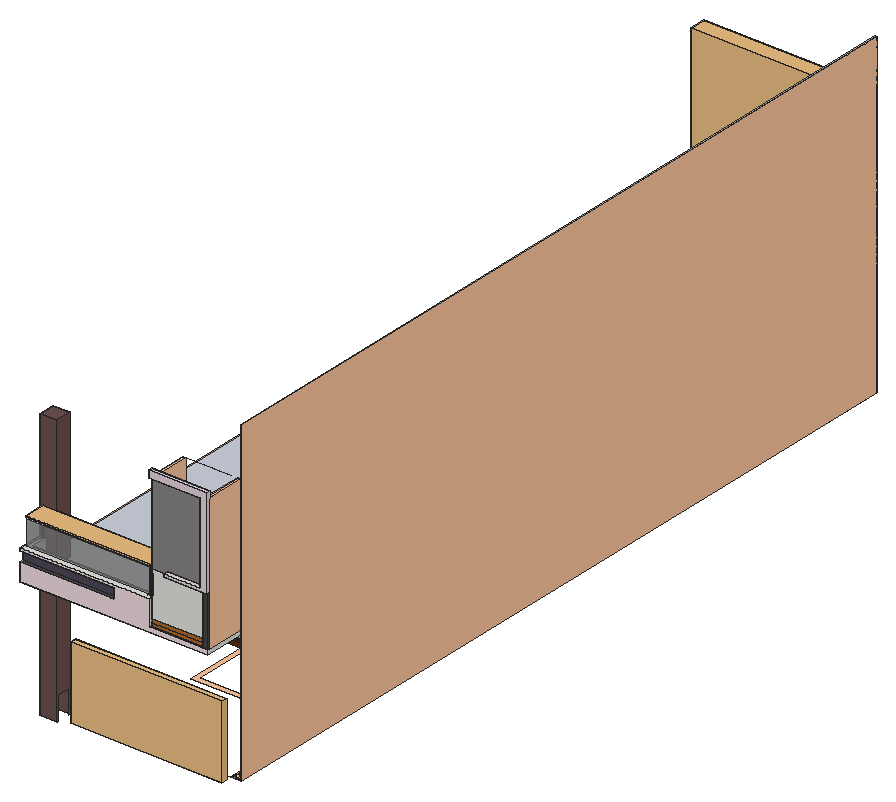
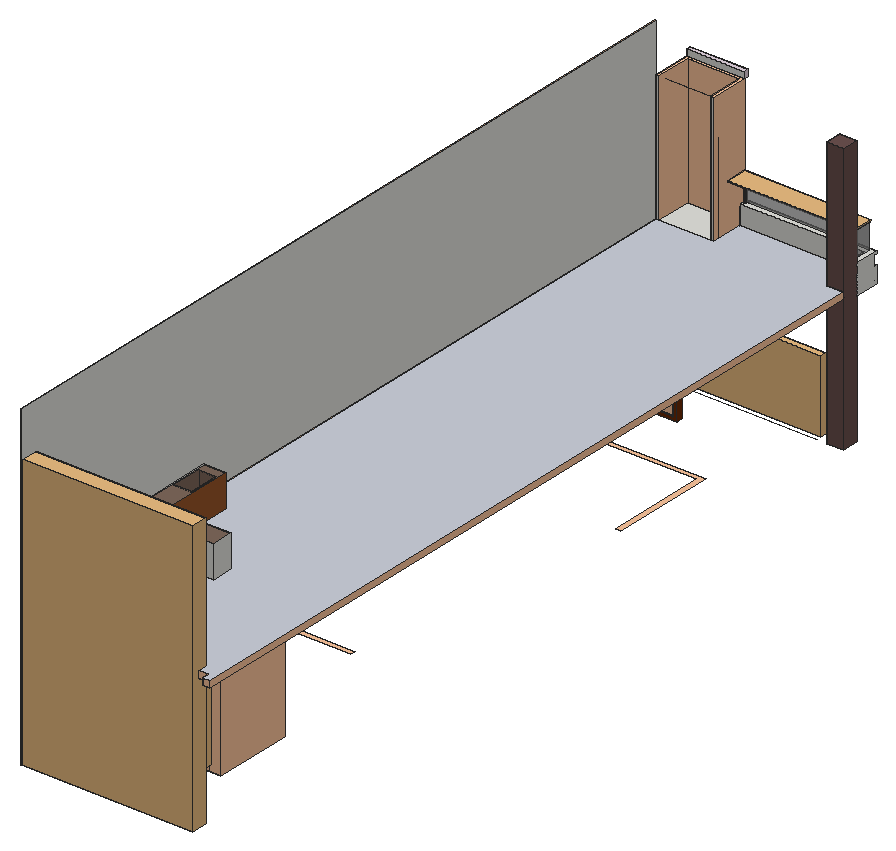
# SketchUp Ruby script. Lengths in inches.
U = 1.inch
M = Sketchup.active_model
def pt(a) = Geom::Point3d.new(a.map { |v| v * U })
def face(e, loops, mat)
  f = e.add_face(loops[0].map { |a| pt(a) })
  loops[1..].each { |l| e.add_face(l.map { |a| pt(a) }).erase! }
  f.material = f.back_material = mat if mat
  f
end
# faces: each face lists its corners as indices into pts; further lists are holes
def faces(e, pts, list, mat = nil) = list.each { |f| face(e, (f[0].is_a?(Array) ? f : [f]).map { |l| l.map { |i| pts[i] } }, mat) }
# xy, xz, yz: faces in a plane at the given z, y or x. An outline is a flat list of corners, or four numbers for a rectangle; further outlines are holes
def ring(l) = l.size == 4 ? [[l[0], l[1]], [l[2], l[1]], [l[2], l[3]], [l[0], l[3]]] : l.each_slice(2).to_a
def flat(e, list, mat, &to3) = list.each { |f| face(e, (f[0].is_a?(Array) ? f : [f]).map { |l| ring(l).map { |u, v| to3.(u, v) } }, mat) }
def xy(e, z, list, mat = nil) = flat(e, list, mat) { |x, y| [x, y, z] }
def xz(e, y, list, mat = nil) = flat(e, list, mat) { |x, z| [x, y, z] }
def yz(e, x, list, mat = nil) = flat(e, list, mat) { |y, z| [x, y, z] }
def lines(e, pts, list) = list.each { |a, b| e.add_line(pt(pts[a]), pt(pts[b])) }
# prism: a flat outline (further loops are holes) pulled along v
def prism(e, loops, v, mat = nil)
  f = face(e, loops, mat); d = Geom::Vector3d.new(v.map { |x| x * U })
  f.pushpull(f.normal.samedirection?(d) ? d.length : -d.length)
end
def box(e, o, s, mat = nil) = prism(e, [[o, [o[0] + s[0], o[1], o[2]], [o[0] + s[0], o[1] + s[1], o[2]], [o[0], o[1] + s[1], o[2]]]], [0, 0, s[2]], mat)
def at(x, y, z, deg = 0) = Geom::Transformation.translation(pt([x, y, z])) * Geom::Transformation.rotation(ORIGIN, Z_AXIS, deg.degrees)
def axes(o, x, y, z) = Geom::Transformation.new([*x, 0, *y, 0, *z, 0, *pt(o).to_a, 1])
def part(name) = M.definitions.add(name)
# library, detail: a bought-in or finely detailed component or shape, given as its bounding box
def library(name, o, s) = part(name).tap { |d| box(d.entities, o, s) }
def detail(e, o, s) = box(e.add_group.entities, o, s)
def put(e, d, t, mat = nil) = e.add_instance(d, t).tap { |i| i.material = mat if mat }
def group(e, t, mat = nil) = e.add_group.tap { |g| g.transformation = t; g.material = mat if mat }.entities
root = M.entities
M.materials.add("[Brick Tumbled]").color = [135, 132, 132]
M.materials.add("[Color A01]").color = [243, 201, 104]
M.materials.add("[Color A02]1").color = [252, 197, 157]
M.materials.add("[Color A02]3").color = [226, 211, 222]
M.materials.add("[Color B01]").color = [107, 81, 79]
M.materials.add("[Color B06]").color = [239, 219, 223]
M.materials.add("[Color M06]").color = [77, 72, 86]
M.materials.add("[Granite Brown]").color = [126, 104, 91]
M.materials.add("[Granite Dark Gray]").color = [69, 68, 68]
M.materials.add("[Marble Carrara Floor Tile]").color = [204, 208, 219]
M.materials.add("[Metal Aluminum Anodized]").color = [202, 209, 219]
M.materials.add("[Tile Veriegated Stone]").color = [171, 137, 112]
M.materials.add("[Translucent Glass Gray]1").color = [132, 132, 132]
M.materials["[Translucent Glass Gray]1"].alpha = 0.5
M.materials.add("[Wood Bamboo]").color = [177, 105, 43]
M.materials.add("[Wood Cherry Original]").color = [152, 86, 42]
M.materials.add("[Wood Fence]").color = [130, 51, 1]
M.materials.add("[Wood Veneer 02]").color = [107, 42, 7]
c1 = library("Group\#155",[-46.99,0,0],[159.06,15.07,255.07])
c2 = library("Slatted double gate",[-0.09,68.76,-0.1],[107.6,5.32,60.06])
c3 = library("Group\#179",[-0.01,-1.53,0.79],[112.05,69.48,120])
c4 = part("Group222\#1")
xy(c4.entities,0,[[[-24,-24,24,24],[-20.4375,-20.4375,-7.1,20.4375],[-6.67,-20.4375,6.67,20.4375],[7.1,-20.4375,20.4375,20.4375]]],"[Wood Veneer 02]")
xy(c4.entities,0.375,[[-20.4375,-20.4375,-20.0625,-20.0625,-7.48,-20.0625,-7.1,-20.4375],[-20.4375,-20.4375,-20.4375,20.4375,-20.0625,20.0625,-20.0625,-20.0625],[-7.1,-20.4375,-7.48,-20.0625,-7.48,20.0625,-7.1,20.4375],[-6.67,-20.4375,-6.29,-20.0625,6.29,-20.0625,6.67,-20.4375],[-6.67,-20.4375,-6.67,20.4375,-6.29,20.0625,-6.29,-20.0625],
  [6.67,-20.4375,6.29,-20.0625,6.29,20.0625,6.67,20.4375],[7.1,-20.4375,7.1,20.4375,7.48,20.0625,7.48,-20.0625],[7.1,-20.4375,7.48,-20.0625,20.0625,-20.0625,20.4375,-20.4375],[20.4375,-20.4375,20.0625,-20.0625,20.0625,20.0625,20.4375,20.4375],[-20.0625,20.0625,-20.4375,20.4375,-7.1,20.4375,-7.48,20.0625],
  [-6.29,20.0625,-6.67,20.4375,6.67,20.4375,6.29,20.0625],[7.48,20.0625,7.1,20.4375,20.4375,20.4375,20.0625,20.0625]],"[Wood Veneer 02]")
xy(c4.entities,5.5,[[-20.4375,-20.4375,-20.0625,-20.0625,-20.0625,20.0625,-20.4375,20.4375],[-20.4375,-20.4375,-7.1,-20.4375,-7.48,-20.0625,-20.0625,-20.0625],[-7.1,-20.4375,-7.1,20.4375,-7.48,20.0625,-7.48,-20.0625],[-6.67,-20.4375,-6.29,-20.0625,-6.29,20.0625,-6.67,20.4375],[-6.67,-20.4375,6.67,-20.4375,6.29,-20.0625,-6.29,-20.0625],
  [6.67,-20.4375,6.67,20.4375,6.29,20.0625,6.29,-20.0625],[7.1,-20.4375,20.4375,-20.4375,20.0625,-20.0625,7.48,-20.0625],[7.1,-20.4375,7.48,-20.0625,7.48,20.0625,7.1,20.4375],[20.4375,-20.4375,20.4375,20.4375,20.0625,20.0625,20.0625,-20.0625],[-20.0625,20.0625,-7.48,20.0625,-7.1,20.4375,-20.4375,20.4375],
  [-6.29,20.0625,6.29,20.0625,6.67,20.4375,-6.67,20.4375],[7.48,20.0625,20.0625,20.0625,20.4375,20.4375,7.1,20.4375]],"[Wood Veneer 02]")
xy(c4.entities,5.875,[[[-24,-24,24,24],[-20.4375,-20.4375,-7.1,20.4375],[-6.67,-20.4375,6.67,20.4375],[7.1,-20.4375,20.4375,20.4375]]],"[Wood Veneer 02]")
xz(c4.entities,-24,[[-24,0,24,5.875]],"[Wood Veneer 02]")
xz(c4.entities,-20.4375,[[-20.4375,0,-7.1,0.375],[-6.67,0,6.67,0.375],[7.1,0,20.4375,0.375],[-20.4375,5.5,-7.1,5.875],[-6.67,5.5,6.67,5.875],
  [7.1,5.5,20.4375,5.875]],"[Wood Veneer 02]")
xz(c4.entities,-20.0625,[[-20.0625,0.375,-7.48,5.5],[-6.29,0.375,6.29,5.5],[7.48,0.375,20.0625,5.5]],"[Wood Veneer 02]")
xz(c4.entities,20.0625,[[-20.0625,0.375,-7.48,5.5],[-6.29,0.375,6.29,5.5],[7.48,0.375,20.0625,5.5]],"[Wood Veneer 02]")
xz(c4.entities,20.4375,[[-20.4375,0,-7.1,0.375],[-6.67,0,6.67,0.375],[7.1,0,20.4375,0.375],[-20.4375,5.5,-7.1,5.875],[-6.67,5.5,6.67,5.875],
  [7.1,5.5,20.4375,5.875]],"[Wood Veneer 02]")
xz(c4.entities,24,[[-24,0,24,5.875]],"[Wood Veneer 02]")
yz(c4.entities,-24,[[-24,0,24,5.875]],"[Wood Veneer 02]")
yz(c4.entities,-20.4375,[[-20.4375,0,20.4375,0.375],[-20.4375,5.5,20.4375,5.875]],"[Wood Veneer 02]")
yz(c4.entities,-20.0625,[[-20.0625,0.375,20.0625,5.5]],"[Wood Veneer 02]")
yz(c4.entities,-7.48,[[-20.0625,0.375,20.0625,5.5]],"[Wood Veneer 02]")
yz(c4.entities,-7.1,[[-20.4375,0,20.4375,0.375],[-20.4375,5.5,20.4375,5.875]],"[Wood Veneer 02]")
yz(c4.entities,-6.67,[[-20.4375,0,20.4375,0.375],[-20.4375,5.5,20.4375,5.875]],"[Wood Veneer 02]")
yz(c4.entities,-6.29,[[-20.0625,0.375,20.0625,5.5]],"[Wood Veneer 02]")
yz(c4.entities,6.29,[[-20.0625,0.375,20.0625,5.5]],"[Wood Veneer 02]")
yz(c4.entities,6.67,[[-20.4375,0,20.4375,0.375],[-20.4375,5.5,20.4375,5.875]],"[Wood Veneer 02]")
yz(c4.entities,7.1,[[-20.4375,0,20.4375,0.375],[-20.4375,5.5,20.4375,5.875]],"[Wood Veneer 02]")
yz(c4.entities,7.48,[[-20.0625,0.375,20.0625,5.5]],"[Wood Veneer 02]")
yz(c4.entities,20.0625,[[-20.0625,0.375,20.0625,5.5]],"[Wood Veneer 02]")
yz(c4.entities,20.4375,[[-20.4375,0,20.4375,0.375],[-20.4375,5.5,20.4375,5.875]],"[Wood Veneer 02]")
yz(c4.entities,24,[[-24,0,24,5.875]],"[Wood Veneer 02]")
c5 = part("Round rod")
prism(c5.entities,[[[1.59,1.03,0],[1.625,0.82,0],[1.6,0.61,0],[1.52,0.42,0],[1.4,0.25,0],[1.23,0.11,0],[1.03,0.03,0],[0.82,0,0],[0.61,0.02,0],[0.42,0.1,0],[0.25,0.23,0],[0.11,0.4,0],[0.03,0.59,0],[0,0.8,0],[0.02,1.01,0],[0.1,1.21,0],[0.23,1.38,0],[0.4,1.51,0],[0.59,1.59,0],[0.8,1.625,0],[1.01,1.6,0],[1.21,1.52,0],[1.38,1.4,0],[1.51,1.23,0]]],[0,0,25.375])
c6 = part("Component\#5")
box(c6.entities,[0,-0.625,0],[48.6875,0.625,3.09])
xy(root,-0.11,[[[166.9,46.0625,175.89,46.0625,175.89,61,171.33,61,171.33,61.13,166.9,61.13],[167.91,47.08,167.91,49.86,168.54,49.23,167.91,48.6,167.91,48.09,168.54,47.46,168.17,47.08,168.93,47.08,168.54,47.46,169.42,48.35,170.32,47.46,169.94,47.08,170.7,47.08,170.32,47.46,171.19,48.36,172.09,47.46,171.71,47.08,172.47,47.08,172.09,47.46,172.95,48.37,172.07,49.26,172.94,50.15,172.06,51.04,171.18,50.14,170.3,51.02,169.42,50.13,170.3,49.25,169.42,48.35,168.54,49.23,169.42,50.13,168.54,51.01,169.42,51.9,168.54,52.78,169.42,53.67,168.54,54.55,167.91,53.91,167.91,53.41,168.54,52.78,167.91,52.14,167.91,58.73,168.55,58.09,169.43,58.98,168.29,60.12,172.35,60.12,170.32,58.09,169.43,58.98,168.55,58.09,169.43,57.21,168.55,56.32,170.3,54.57,171.18,55.46,172.06,56.36,172.93,55.48,173.8125,56.37,172.93,57.25,173.8125,58.15,174.69,59.04,173.8,59.93,173.99,60.12,174.88,60.12,174.88,59.23,174.69,59.04,173.8125,58.15,174.69,57.27,173.8125,56.37,174.69,55.49,174.88,55.31,174.88,53.91,174.69,53.72,173.8125,52.83,172.93,51.93,173.82,51.05,174.69,50.17,172.95,48.37,173.85,47.47,173.49,47.08],[174.88,57.08,174.69,57.27,174.88,57.46],[174.88,48.22,174.7,48.4,174.88,48.6]],[167.91,47.08,168.17,47.08,168.54,47.46,167.91,48.09],[168.93,47.08,169.94,47.08,170.32,47.46,169.42,48.35,168.54,47.46],[170.7,47.08,171.71,47.08,172.09,47.46,171.19,48.36,170.32,47.46],[172.47,47.08,173.49,47.08,173.85,47.47,172.95,48.37,172.09,47.46],
  [174.25,47.08,174.88,47.08,174.88,48.22,174.7,48.4,173.85,47.47],[174.88,48.22,174.88,48.6,174.7,48.4],[167.91,48.6,168.54,49.23,167.91,49.86],[174.88,49.99,174.88,50.37,174.69,50.17],[167.91,50.37,168.54,51.01,167.91,51.63],
  [174.88,51.76,174.88,52.14,174.69,51.95],[171.18,51.92,172.06,52.8125,172.93,53.71,170.3,56.34,169.42,55.45,168.55,56.32,167.91,55.6875,167.91,55.18,169.42,53.67,170.3,52.8],[167.91,52.14,168.54,52.78,167.91,53.41],[174.69,53.72,174.88,53.91,174.88,55.31,174.69,55.49,173.8125,54.6],[167.91,53.91,168.54,54.55,167.91,55.18],
  [167.91,55.6875,168.55,56.32,167.91,56.95],[168.55,56.32,167.91,56.95,167.91,57.46,168.55,58.09,170.3,56.34,171.17,57.24,170.32,58.09,169.43,57.21],[174.88,57.08,174.88,57.46,174.69,57.27],[167.91,57.46,168.55,58.09,167.91,58.73],[174.69,59.04,174.88,59.23,174.88,60.12,173.99,60.12,173.8,59.93],
  [168.55,59.86,168.8,60.12,168.29,60.12],[170.32,59.86,170.57,60.12,170.07,60.12],[172.09,59.86,172.35,60.12,171.84,60.12],[171.33,61,175.89,61.13],[171.33,61.13,171.33,142.17,142.65,142.17,141.07,143.82,140.6875,143.4375,142.01,142.17,52.81,142.17,52.81,241.2,57.37,241.2,57.37,146.61,171.33,146.61,171.33,212.2,175.89,212.2,175.89,61.13],
  [142.01,142.17,140.6875,143.4375,141.07,143.82,142.65,142.17],[166.9,212.2,171.33,212.2,171.33,213.21,167.91,213.21,167.91,226.13,171.33,226.13,171.33,227.14,166.9,227.14],[171.33,212.2,175.89,212.2,175.89,227.14,171.33,227.14,171.33,226.13,174.88,226.13,174.88,213.21,171.33,213.21],[167.91,213.21,168.17,213.21,168.55,213.59,167.91,214.22],[168.17,213.21,168.93,213.21,168.55,213.59],
  [168.93,213.21,169.94,213.21,170.32,213.59,169.43,214.48,168.55,213.59],[169.94,213.21,170.7,213.21,170.32,213.59],[170.7,213.21,171.33,213.21,171.33,214.35,171.21,214.48,170.32,213.59],[171.33,213.21,171.71,213.21,172.09,213.59,171.33,214.35],[172.47,213.21,173.49,213.21,173.87,213.59,172.98,214.48,172.09,213.59],
  [170.32,213.59,171.21,214.48,170.32,215.36,169.43,214.48],[174.88,214.22,174.88,214.6,174.69,214.42],[174.69,214.42,174.88,214.6,174.88,216,174.69,216.1875,173.8125,215.3125],[171.33,214.6,172.09,215.36,171.33,216.125],[171.33,216.125,171.33,216.38,171.21,216.25],
  [171.33,216.38,172.06,217.1,171.33,217.83],[172.06,217.1,172.93,217.98,172.06,218.87,171.33,218.15,171.33,217.83],[171.33,217.83,171.33,218.15,171.18,217.99],[169.43,218.02,170.3,218.89,169.42,219.78,168.55,218.91],[171.33,218.15,172.06,218.87,171.33,219.61],
  [172.06,218.87,172.92,219.73,172.03,220.62,171.33,219.92,171.33,219.61],[170.3,218.89,171.18,219.77,170.3,220.66,169.42,219.78],[171.33,219.61,171.33,219.92,171.18,219.77],[169.42,219.78,170.3,220.66,169.42,221.56,168.54,220.68],[172.03,220.62,172.92,221.51,172.03,222.39,171.33,221.7,171.33,221.32],
  [173.8,220.62,174.6875,221.51,173.8,222.39,172.92,221.51],[170.3,220.66,171.14,221.51,170.26,222.39,169.42,221.56],[171.33,221.32,171.33,221.7,171.14,221.51],[171.14,221.51,171.33,221.7,171.33,223.09,171.14,223.28,170.26,222.39],[172.92,221.51,173.8,222.39,172.92,223.28,172.03,222.39],
  [172.03,222.39,172.92,223.28,172.03,224.16,171.33,223.47,171.33,223.09],[173.8,222.39,174.6875,223.28,173.8,224.16,172.92,223.28],[171.33,223.09,171.33,223.47,171.14,223.28],[169.39,223.26,170.29,224.13,169.41,225.02,168.5,224.15],[172.92,223.28,173.8,224.16,172.92,225.05,172.03,224.16],
  [167.91,223.6,168.5,224.15,167.91,224.73],[170.29,224.13,171.19,225,170.3125,225.88,169.41,225.02],[168.5,224.15,169.41,225.02,168.53,225.89,167.91,225.37,167.91,224.73],[173.8,224.16,174.6875,225.05,173.8,225.9375,172.92,225.05],[168.17,372.26,168.93,372.26,168.55,372.64],
  [171.33,372.26,171.71,372.26,172.09,372.64,171.33,373.4],[171.71,372.26,172.47,372.26,172.09,372.64],[169.43,373.52,170.32,374.41,169.43,375.3,168.55,374.41],[170.32,374.41,171.21,375.3,170.32,376.18,169.43,375.3],[169.43,375.3,170.32,376.18,169.43,377.07,168.55,376.18],
  [171.21,375.3,171.33,375.42,171.33,376.88,171.18,377.04,170.32,376.18],[170.32,376.18,171.18,377.04,170.3,377.93,169.43,377.07],[174.88,376.82,174.88,377.19,174.69,377.01],[174.69,377.01,174.88,377.19,174.88,378.59,174.69,378.78,173.8125,377.9],[169.43,377.07,170.3,377.93,169.42,378.83,168.55,377.95],
  [170.3,377.93,171.18,378.8125,170.3,379.71,169.42,378.83],[174.69,378.78,174.88,378.97,174.88,380.36,174.69,380.55,173.8125,379.67],[169.42,378.83,170.3,379.71,169.4,380.62,168.53,379.73],[170.3,379.71,171.18,380.58,170.27,381.5,169.4,380.62],[174.69,380.55,174.88,380.74,174.88,382.13,174.69,382.33,173.82,381.45],
  [169.4,380.62,170.27,381.5,169.42,382.37,168.54,381.49],[170.27,381.5,171.15,382.39,170.3,383.25,169.42,382.37],[172.94,382.35,173.82,383.23,172.9,384.1875,172.02,383.29],[169.42,382.37,170.3,383.25,169.42,384.15,168.54,383.27],[173.82,383.23,174.7,384.11,173.8,385.1,172.9,384.1875],
  [170.3,383.25,171.19,384.14,170.32,385.04,169.42,384.15],[173.8,385.1,173.99,385.3,173.61,385.3],[171.33,386.1875,171.33,501.8,92.32,501.8,92.32,506.23,171.33,506.23,171.33,563.34,175.89,563.34,175.89,386.1875],[166.9,563.34,175.89,563.34,175.89,578.28,171.33,578.28,171.33,577.27,174.88,577.27,174.88,564.35,167.91,564.35,167.91,577.27,171.33,577.27,171.33,578.28,166.9,578.28],[167.91,564.35,168.17,564.35,168.55,564.73,167.91,565.36],
  [168.17,564.35,168.93,564.35,168.55,564.73,169.43,565.62,168.55,566.5,167.91,565.87,167.91,565.36,168.55,564.73],[169.94,564.35,170.7,564.35,170.32,564.73],[171.71,564.35,172.47,564.35,172.09,564.73],[172.47,564.35,173.49,564.35,173.87,564.73,172.98,565.62,172.09,564.73],[173.49,564.35,174.25,564.35,173.87,564.73],
  [174.25,564.35,174.88,564.35,174.88,565.36,174.69,565.56,173.87,564.73],[168.55,564.73,169.43,565.62,168.55,566.5,167.91,565.87,167.91,565.36],[172.09,564.73,172.98,565.62,172.09,566.5,171.21,565.62],[171.21,565.62,172.09,566.5,171.21,567.39,170.32,566.5],[167.91,565.87,168.55,566.5,167.91,567.14],
  [168.55,566.5,169.43,567.39,168.55,568.28,167.91,567.64,167.91,567.14],[172.09,566.5,172.93,567.34,172.06,568.24,171.21,567.39],[167.91,567.64,168.55,568.28,167.91,568.91],[168.55,568.28,169.43,569.16,168.55,570.05,167.91,569.42,167.91,568.91],[174.88,568.91,174.88,569.29,174.6875,569.1],
  [171.33,568.97,171.33,569.29,171.18,569.13],[174.6875,569.1,174.88,569.29,174.88,570.68,174.6875,570.87,173.8,569.99],[173.8,571.76,174.6875,572.65,173.8,573.53,172.92,572.65],[172.92,572.65,173.8,573.53,172.92,574.42,172.03,573.53],[172.03,573.53,172.92,574.42,172.03,575.3,171.33,574.61,171.33,574.23],
  [173.8,573.53,174.6875,574.42,173.8,575.3,172.92,574.42],[171.33,574.23,171.33,574.61,171.14,574.42],[174.88,574.23,174.88,574.61,174.6875,574.42],[172.92,574.42,173.8,575.3,172.92,576.19,172.03,575.3],[172.03,575.3,172.92,576.19,172.09,577.02,171.33,576.28,171.33,576],
  [173.8,575.3,174.6875,576.19,173.8,577.08,172.92,576.19],[172.92,576.19,173.8,577.08,173.61,577.27,172.35,577.27,172.09,577.02],[174.6875,576.19,174.88,576.38,174.88,577.27,173.99,577.27,173.8,577.08],[171.33,576.28,172.09,577.02,171.84,577.27,171.33,577.27],[172.09,577.02,172.35,577.27,171.84,577.27],
  [173.8,577.08,173.99,577.27,173.61,577.27],[171.33,578.28,175.89,578.28,175.89,706.3,52.81,706.3,52.81,632.35,57.37,632.35,57.37,637.29,69.4,637.29,69.4,641.85,57.37,641.85,57.37,701.87,171.33,701.87],[89.4,637.29,171.33,641.85]],"[Color A02]1")
xy(root,0,[[175.91,46.0625,175.89,785.32,176.89,785.32,176.91,46.0625]])
xy(root,113.57,[[153.02,587.14,169.46,615.87]],"[Granite Brown]")
xy(root,125.89,[[0.89,46.0625,7.86,784.43],[171.33,61,175.89,61,175.89,212.2,171.33,212.2,171.33,146.61,57.37,146.61,57.37,241.2,52.81,241.2,52.81,142.17,142.01,142.17,140.6875,143.4375,141.07,143.82,142.65,142.17,171.33,142.17],[142.01,142.17,142.26,142.17,140.6875,143.4375],[142.26,142.17,142.65,142.17,141.07,143.82,140.6875,143.4375],[171.33,227.14,175.89,227.14,175.89,371.24,171.33,371.24,171.33,318.69,126.89,318.69,126.89,341.23,122.33,341.23,122.33,318.69,57.37,318.69,57.37,371.24,126.89,371.24,126.89,375.68,57.37,375.68,57.37,501.8,63.32,501.8,63.32,506.23,57.37,506.23,57.37,585.88,52.81,585.88,52.81,283.24,57.37,283.24,57.37,314.26,171.33,314.26],
  [171.33,386.1875,175.89,386.1875,175.89,563.34,171.33,563.34,171.33,506.23,92.32,506.23,92.32,501.8,171.33,501.8],[171.33,578.28,175.89,578.28,175.89,706.3,52.81,706.3,52.81,632.35,57.37,632.35,57.37,637.29,69.4,637.29,69.4,641.85,57.37,641.85,57.37,701.87,171.33,701.87]],"[Color A02]1")
xy(root,131.89,[[151.27,578.28,151.27,646.1,92.44,646.1,92.44,665.91,171.33,665.91,171.33,578.28]])
xy(root,161.89,[[[151.27,578.28,171.33,578.28,171.33,665.91,92.44,665.91,92.44,646.1,151.27,646.1],[153.02,587.14,169.46,615.87]]],"[Granite Brown]")
xy(root,297.2,[[175.91,46.0625,176.91,46.0625,176.89,785.32,175.89,785.32]])
xz(root,46.0625,[[175.91,0,176.91,297.2]])
xz(root,61,[[171.33,-0.11,175.89,125.89]],"[Color A02]1")
xz(root,146.61,[[75.18,41.89,123.18,89.89]],"[Color A02]1")
xz(root,212.2,[[166.89,125.89,175.89,125.9]],"[Color A02]1")
xz(root,227.14,[[166.89,125.89,175.89,125.9]],"[Color A02]1")
xz(root,371.25,[[166.89,125.89,175.89,125.9]],"[Color A02]1")
xz(root,386.1875,[[166.89,125.89,175.89,125.9]],"[Color A02]1")
xz(root,563.34,[[173.33,125.89,175.89,125.9]],"[Color A02]1")
xz(root,578.28,[[151.27,131.89,171.33,161.89]])
xz(root,578.28,[[171.33,-0.11,175.89,125.89],[166.7,125.89,166.9,125.9],[173.33,125.89,175.89,125.9]],"[Color A02]1")
xz(root,587.14,[[153.02,113.57,169.46,161.89]],"[Granite Brown]")
xz(root,615.87,[[153.02,113.57,169.46,161.89]],"[Granite Brown]")
xz(root,632.35,[[52.81,-0.11,57.37,125.89]],"[Color A02]1")
xz(root,637.29,[[57.37,-0.11,69.4,125.89]],"[Color A02]1")
xz(root,641.85,[[57.37,-0.11,69.4,125.89]],"[Color A02]1")
xz(root,646.1,[[92.44,131.89,151.27,161.89]],"[Wood Cherry Original]")
xz(root,665.91,[[92.44,131.89,171.33,161.89]])
xz(root,701.87,[[57.37,-0.11,171.33,0],[57.37,0,171.33,125.89],[171.33,0,171.91,125.89]],"[Color A02]1")
xz(root,706.3,[[52.81,-0.11,63.83,125.89],[63.83,-0.11,73.83,125.89],[73.83,-0.11,83.83,125.89],[83.83,-0.11,93.84,125.89],[93.84,-0.11,103.84,125.89],
  [103.84,-0.11,113.84,125.89],[113.84,-0.11,123.85,125.89],[123.85,-0.11,133.85,125.89],[133.85,-0.11,175.89,125.89]],"[Color A02]1")
xz(root,785.32,[[175.89,0,176.89,257.89],[175.89,257.89,176.89,297.2]])
yz(root,52.81,[[632.35,-0.11,706.3,125.89]],"[Color A02]1")
yz(root,57.37,[[632.35,-0.11,637.29,125.89],[641.85,-0.11,677.81,125.89],[677.81,-0.11,701.87,125.89]],"[Color A02]1")
yz(root,69.4,[[637.29,-0.11,641.85,125.89]],"[Color A02]1")
yz(root,92.44,[[646.1,131.89,665.91,161.89]])
yz(root,151.27,[[578.28,131.89,646.1,161.89]],"[Wood Cherry Original]")
yz(root,153.02,[[587.14,113.57,615.87,161.89]],"[Granite Brown]")
yz(root,166.89,[[212.2,125.89,227.14,125.9],[371.25,125.89,386.1875,125.9]],"[Color A02]1")
yz(root,169.46,[[587.14,113.57,615.87,161.89]],"[Granite Brown]")
yz(root,171.33,[[578.28,131.89,665.91,161.89]])
yz(root,171.33,[[61,-0.11,142.17,125.89],[578.28,-0.11,677.81,125.89],[677.81,-0.11,701.87,125.89]],"[Color A02]1")
yz(root,175.89,[[578.28,-0.11,706.3,125.89],[227.14,125.89,371.25,125.9],[386.1875,125.89,563.34,125.9]],"[Color A02]1")
p = [[175.89,785.32,257.89],[175.89,785.32,0],[175.91,46.0625,0],[175.91,46.0625,297.2],[175.89,785.32,297.2],[176.89,785.32,0],
  [176.89,785.32,257.89],[176.89,785.32,297.2],[176.91,46.0625,297.2],[176.91,46.0625,0],[25.85,46.0625,0],[166.9,46.0625,0],
  [166.9,61,121.89],[166.9,58.0625,121.89],[166.91,769.5,60],[166.91,769.76,60],[0.89,10.0625,125.89],[0.89,10.0625,125.9],
  [0.89,784.43,125.89],[0.89,784.43,125.9],[175.89,784.43,125.89],[175.89,784.43,125.9],[175.89,10.0625,125.89],[175.89,10.0625,125.9],
  [175.89,61,125.89],[175.89,46.0625,125.89],[92.89,146.61,45.82],[92.89,146.61,85.95],[79.12,146.61,85.95],[91.7,146.61,85.95],
  [79.12,146.61,45.82],[105.48,146.61,45.82],[91.7,146.61,45.82],[105.48,146.61,85.95],[106.66,146.61,45.82],[106.66,146.61,85.95],
  [119.25,146.61,45.82],[119.25,146.61,85.95],[91.7,145.11,45.82],[79.12,145.11,45.82],[79.12,145.11,85.95],[91.7,145.11,85.95],
  [105.48,145.11,45.82],[92.89,145.11,45.82],[92.89,145.11,85.95],[105.48,145.11,85.95],[119.25,145.11,45.82],[106.66,145.11,45.82],
  [106.66,145.11,85.95],[119.25,145.11,85.95]]
faces(root,p,[[0,1,2,3,4]])
faces(root,p,[[5,6,7,8,9]],"[Color A02]1")
lines(root,p,[[10,11],[12,13],[14,15],[16,17],[18,19],[20,21],[22,23],[24,25],[26,27],[28,29],[30,28],[31,26],
  [32,30],[27,33],[29,32],[33,31],[34,35],[36,34],[37,36],[35,37],[38,39],[39,40],[40,41],[41,38],
  [42,43],[43,44],[44,45],[45,42],[46,47],[47,48],[48,49],[49,46]])
put(root,c1,at(63.84,769.36,0))
g1 = group(root,at(0.89,30.95,0))
xy(g1,251.89,[[0,0,15.96,15.11]],"[Color B01]")
xz(g1,0,[[0,0,15.96,251.89]],"[Color B01]")
xz(g1,15.11,[[0,0,15.96,251.89]],"[Color B01]")
yz(g1,0,[[0,0,15.11,251.89]],"[Color B01]")
yz(g1,15.96,[[0,0,0.84,0,0.84,21.875,13.375,21.875,13.375,0,15.11,0,15.11,251.89,0,251.89]],"[Color B01]")
put(root,c2,axes([25.96,-33.09,0.11],[1.31104,0,0],[0,1,0],[0,0,1.1312]))
put(root,c3,at(62.29,707.83,5.1))
put(root,c4,axes([99.18,148.05,65.89],[1,0,0],[0,0,1],[0,-1,0]),"[Color A02]1")
g2 = group(root,at(0.89,46.0625,125.89))
xy(g2,-1.5625,[[26.98,-0.11,153.05,81.35]],"[Wood Fence]")
xy(g2,0,[[169.6875,-38,175,-36],[[6.97,-20.12,6.97,-15.11,15.96,-15.11,15.96,0,6.97,0,6.97,101.35,173.05,101.35,173.05,-20.12],[26.98,-0.11,153.05,81.35]],[6.97,-15.11,15.96,0]])
xy(g2,0,[[121,-36,121,-31.625,4.5,-31.625,4.5,-15.11,6.97,-15.11,6.97,-20.12,173.05,-20.12,173.05,101.35,6.97,101.35,6.97,0,0,0,0,738.37,6.96,738.37,6.96,732.29,61.39,732.29,61.39,698.9,173.47,698.9,173.47,660.17,175,660.17,175,-36]],"[Color A02]1")
xy(g2,6,[[124,-33,172,0]])
xy(g2,6,[[4.5,-31.5,121,-31.5,121,0,175,0,175,660.17,173.47,660.17,173.47,698.9,61.39,698.9,61.39,732.29,6.96,732.29,6.96,738.37,0,738.37,0,0,15.96,0,15.96,-15.11,4.5,-15.11]],"[Marble Carrara Floor Tile]")
xy(g2,47.9375,[[135.5625,-40,169.6875,-36],[169.6875,-40,175,-38],[169.6875,-38,175,-36]])
xy(g2,50.9375,[[135.5625,-40,169,-36]],"[Color A02]3")
xy(g2,126,[[121,-40,169,-36]])
xy(g2,126,[[121,-36,175,-36,175,0,172,0,172,-33,124,-33,124,0,121,0]],"[Color A02]1")
xy(g2,132,[[121,-40,175,-36]],"[Color A02]3")
xz(g2,-40,[[135.5625,47.9375,175,47.9375,175,132,121,132,121,126,169,126,169,50.9375,135.5625,50.9375]],"[Color A02]3")
xz(g2,-38,[[169.6875,0,175,47.9375]],"[Granite Dark Gray]")
xz(g2,-36,[[121,0,169.6875,47.9375],[169.6875,0,175,47.9375],[135.5625,47.9375,135.5625,50.9375,169,50.9375,169,126,175,126,175,47.9375],[121,126,175,132]])
xz(g2,-36,[[121,47.9375,135.5625,47.9375,135.5625,50.9375,169,50.9375,169,126,121,126]],"[Brick Tumbled]")
xz(g2,-33,[[124,6,172,126]],"[Color A02]1")
xz(g2,-31.625,[[4.5,0,121,6]])
xz(g2,-15.11,[[4.5,0,15.96,6]])
xz(g2,-0.11,[[26.98,-1.5625,153.05,0]])
xz(g2,0,[[0,0,0.01,6],[0.01,0,15.96,6],[121,6,124,126],[172,6,175,126]])
xz(g2,81.35,[[26.98,-1.5625,153.05,0]])
xz(g2,660.17,[[173.47,0,175,6]],"[Color A02]1")
xz(g2,698.9,[[61.39,0,173.47,6]],"[Color A02]1")
xz(g2,732.29,[[6.96,0,61.39,6]],"[Color A02]1")
xz(g2,738.37,[[0,0,6.96,6]],"[Color A02]1")
yz(g2,0,[[0,0,738.37,6]],"[Color A02]1")
yz(g2,4.5,[[-31.625,0,-15.11,6]])
yz(g2,6.96,[[732.29,0,738.37,6]],"[Color A02]1")
yz(g2,15.96,[[-15.11,0,0,6]])
yz(g2,26.98,[[-0.11,-1.5625,81.35,0]])
yz(g2,61.39,[[698.9,0,732.29,6]],"[Tile Veriegated Stone]")
yz(g2,121,[[-36,0,-31.625,6]])
yz(g2,121,[[-36,6,0,126]],"[Color A02]1")
yz(g2,121,[[-40,126,-36,132]],"[Color A02]3")
yz(g2,124,[[-33,6,0,126]],"[Color A02]1")
yz(g2,135.5625,[[-40,47.9375,-36,50.9375]])
yz(g2,153.05,[[-0.11,-1.5625,81.35,0]])
yz(g2,169,[[-40,50.9375,-36,126]],"[Color A02]3")
yz(g2,169.6875,[[-38,0,-36,47.9375]],"[Granite Dark Gray]")
yz(g2,172,[[-33,6,0,126]],"[Color A02]1")
yz(g2,173.47,[[660.17,0,698.9,6]],"[Color A02]1")
yz(g2,175,[[-36,0,660.17,0,660.17,6,0,6,0,126,-36,126]],"[Color A02]1")
yz(g2,175,[[-40,47.9375,-36,132]],"[Color A02]3")
yz(g2,175,[[-38,0,-36,47.9375]],"[Granite Dark Gray]")
p = [[175,-33.18,126],[175.01,-33.18,126],[121,-5.375,6],[121,-5.375,90],[121.17,-33.62,47.48],[169.6875,-36,47.9375],
  [124,0,126],[166.01,0,126]]
lines(g2,p,[[0,1],[2,3],[4,5],[6,7]])
detail(g2,[2.64,-34.93,49.18],[117.47,19.82,1.24])
g3 = group(g2,at(0,-36,6))
xy(g3,-10.125,[[0,-2,0,20.89,5.92,20.89,5.92,15.88,166.01,15.88,166.01,36,175,36,175,-2]])
xy(g3,-6,[[121,-2,175,-2,175,36,166.01,36,166.01,15.88,121,15.88],[5.92,5.35,121,15.88]])
xy(g3,6,[[0,-2,87.5625,1.25]],"[Color M06]")
xy(g3,15.625,[[0,-2,87.5625,1.25]],"[Color M06]")
xy(g3,18,[[[0,-2,121,-2,121,5.35,5.92,5.35,5.92,20.89,3.39,20.89,3.39,20.75,3.26,20.75,3.26,20.89,0,20.89],[3.39,1.76,117.61,1.97]]])
xy(g3,42,[[3.39,1.76,117.61,1.97]])
xy(g3,42,[[3.26,1.97,3.39,20.75]],"[Translucent Glass Gray]1")
xz(g3,-2,[[0,-10.125,175,-10.125,175,-6,121,-6,121,18,0,18,0,15.625,87.5625,15.625,87.5625,6,0,6]],"[Color B06]")
xz(g3,1.25,[[0,6,87.5625,15.625]],"[Color M06]")
xz(g3,1.76,[[3.39,18,117.61,42]],"[Translucent Glass Gray]1")
xz(g3,1.97,[[3.26,18,117.61,42]],"[Translucent Glass Gray]1")
xz(g3,5.35,[[5.92,-6,121,18]])
xz(g3,15.88,[[5.92,-10.125,166.01,-6]])
xz(g3,20.75,[[3.26,18,3.39,42]],"[Translucent Glass Gray]1")
xz(g3,20.89,[[0,-10.125,5.92,18]])
xz(g3,36,[[166.01,-10.125,175,-6]])
yz(g3,0,[[-2,-10.125,-2,6,1.25,6,1.25,15.625,-2,15.625,-2,18,20.89,18,20.89,-10.125]])
yz(g3,3.26,[[1.97,18,20.75,42]],"[Translucent Glass Gray]1")
yz(g3,5.92,[[15.88,-10.125,20.89,-10.125,20.89,18,5.35,18,5.35,-6,15.88,-6]])
yz(g3,87.5625,[[-2,6,1.25,15.625]],"[Color M06]")
yz(g3,117.61,[[1.76,18,1.97,42]])
yz(g3,121,[[-2,-6,5.35,18]])
yz(g3,166.01,[[15.88,-10.125,36,-10],[15.88,-10,36,-6]])
yz(g3,175,[[-2,-10.125,36,-6]])
put(g3,c5,at(118.6,0.82,18),"[Metal Aluminum Anodized]")
put(g3,c5,at(2.57,19.57,18),"[Metal Aluminum Anodized]")
g4 = group(root,at(7.87,25.95,125.89))
xy(g4,-4,[[[0,0,0,5,8.99,5,8.99,20.12,0,20.12,0,121.47,166.08,121.47,166.08,32.12,159.04,32.12,159.04,0],[20,20,146.07,101.46]]],"[Color A02]1")
xy(g4,-2.9375,[[20,18,146.07,20]],"[Color A01]")
xy(g4,-2.92,[[146.07,18,148.07,101.46],[20,101.46,148.07,103.46]],"[Color A01]")
xy(g4,-2.75,[[18,18,20,103.46]],"[Color A01]")
xy(g4,0,[[[0,0,159.04,0,159.04,32.12,166.08,32.12,166.08,121.47,0,121.47,0,20.12,8.99,20.12,8.99,5,0,5],[18,18,148.07,103.46]]],"[Color A01]")
xz(g4,0,[[0,-4,159.04,0]],"[Color A01]")
xz(g4,5,[[0,-4,8.99,0]],"[Color A01]")
xz(g4,18,[[20,-2.9375,20,-2.75,18,-2.75,18,0,148.07,0,148.07,-2.92,146.07,-2.92,146.07,-2.9375]],"[Color A01]")
xz(g4,20,[[20,-4,146.07,-2.9375]],"[Color A01]")
xz(g4,20.12,[[0,-4,8.99,0]],"[Color A01]")
xz(g4,32.12,[[159.04,-4,166.08,0]],"[Color A01]")
xz(g4,101.46,[[20,-4,146.07,-2.92]],"[Color A01]")
xz(g4,103.46,[[20,-2.92,148.07,-2.92,148.07,0,18,0,18,-2.75,20,-2.75]],"[Color A01]")
xz(g4,121.47,[[0,-4,166.08,0]],"[Color A01]")
yz(g4,0,[[0,-4,5,0],[20.12,-4,121.47,0]],"[Color A01]")
yz(g4,8.99,[[5,-4,20.12,0]],"[Color A01]")
yz(g4,18,[[18,-2.75,103.46,0]],"[Color A01]")
yz(g4,20,[[20,-4,101.46,-4,101.46,-2.92,103.46,-2.92,103.46,-2.75,18,-2.75,18,-2.9375,20,-2.9375]],"[Color A01]")
yz(g4,146.07,[[20,-4,20,-2.9375,18,-2.9375,18,-2.92,101.46,-2.92,101.46,-4]],"[Color A01]")
yz(g4,148.07,[[18,-2.92,103.46,0]],"[Color A01]")
yz(g4,159.04,[[0,-4,20.12,0],[20.12,-4,32.12,0]],"[Color A01]")
yz(g4,166.08,[[32.12,-4,121.47,0]],"[Color A01]")
put(root,c6,at(121.89,10.0625,126.14),"[Wood Bamboo]")
put(root,c6,at(121.89,10.0625,129.31),"[Wood Bamboo]")
